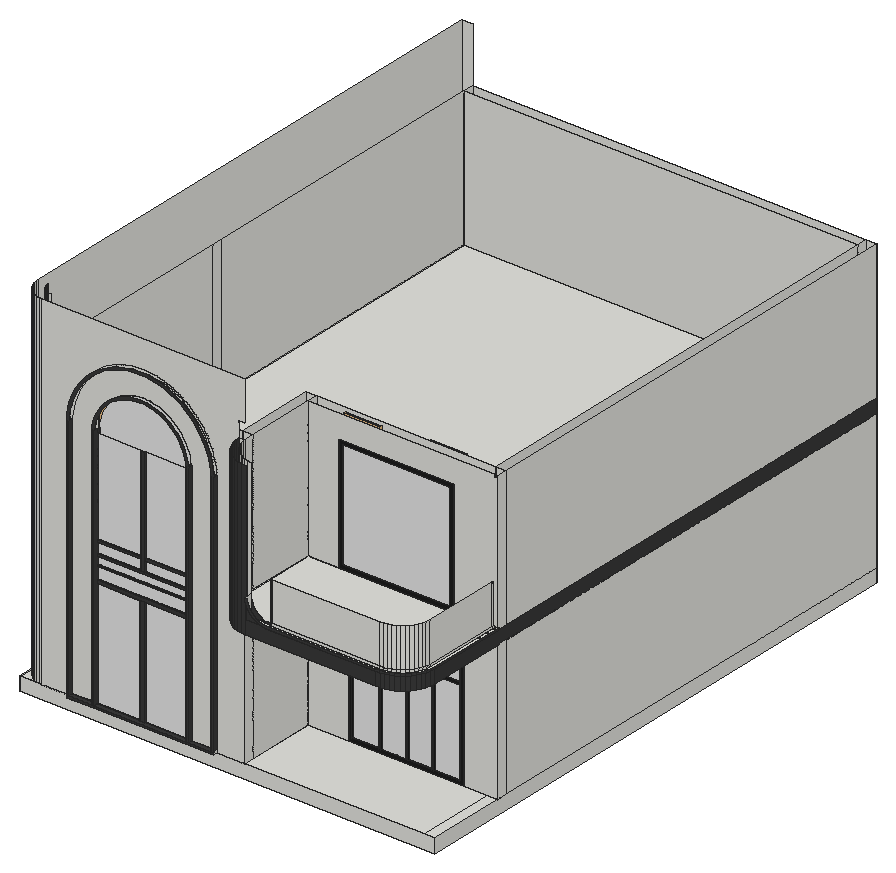
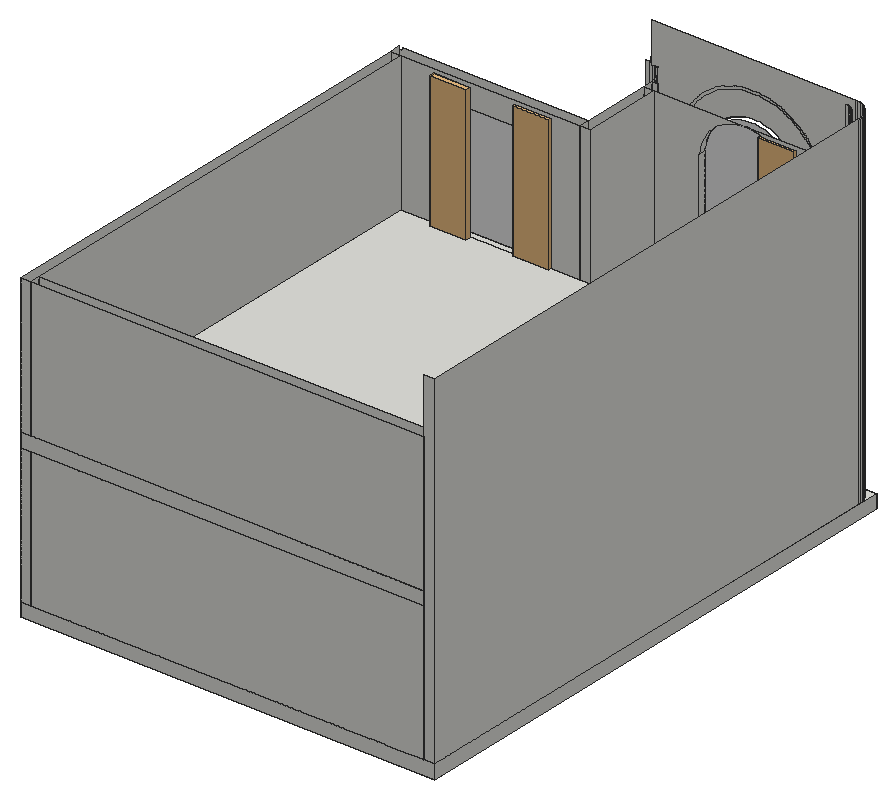
# SketchUp Ruby script. Lengths in inches.
U = 1.inch
M = Sketchup.active_model
def pt(a) = Geom::Point3d.new(a.map { |v| v * U })
def face(e, loops, mat)
  f = e.add_face(loops[0].map { |a| pt(a) })
  loops[1..].each { |l| e.add_face(l.map { |a| pt(a) }).erase! }
  f.material = f.back_material = mat if mat
  f
end
# faces: each face lists its corners as indices into pts; further lists are holes
def faces(e, pts, list, mat = nil) = list.each { |f| face(e, (f[0].is_a?(Array) ? f : [f]).map { |l| l.map { |i| pts[i] } }, mat) }
# xy, xz, yz: faces in a plane at the given z, y or x. An outline is a flat list of corners, or four numbers for a rectangle; further outlines are holes
def ring(l) = l.size == 4 ? [[l[0], l[1]], [l[2], l[1]], [l[2], l[3]], [l[0], l[3]]] : l.each_slice(2).to_a
def flat(e, list, mat, &to3) = list.each { |f| face(e, (f[0].is_a?(Array) ? f : [f]).map { |l| ring(l).map { |u, v| to3.(u, v) } }, mat) }
def xy(e, z, list, mat = nil) = flat(e, list, mat) { |x, y| [x, y, z] }
def xz(e, y, list, mat = nil) = flat(e, list, mat) { |x, z| [x, y, z] }
def yz(e, x, list, mat = nil) = flat(e, list, mat) { |y, z| [x, y, z] }
def lines(e, pts, list) = list.each { |a, b| e.add_line(pt(pts[a]), pt(pts[b])) }
# prism: a flat outline (further loops are holes) pulled along v
def prism(e, loops, v, mat = nil)
  f = face(e, loops, mat); d = Geom::Vector3d.new(v.map { |x| x * U })
  f.pushpull(f.normal.samedirection?(d) ? d.length : -d.length)
end
def box(e, o, s, mat = nil) = prism(e, [[o, [o[0] + s[0], o[1], o[2]], [o[0] + s[0], o[1] + s[1], o[2]], [o[0], o[1] + s[1], o[2]]]], [0, 0, s[2]], mat)
def at(x, y, z, deg = 0) = Geom::Transformation.translation(pt([x, y, z])) * Geom::Transformation.rotation(ORIGIN, Z_AXIS, deg.degrees)
def axes(o, x, y, z) = Geom::Transformation.new([*x, 0, *y, 0, *z, 0, *pt(o).to_a, 1])
def part(name) = M.definitions.add(name)
# library, detail: a bought-in or finely detailed component or shape, given as its bounding box
def library(name, o, s) = part(name).tap { |d| box(d.entities, o, s) }
def detail(e, o, s) = box(e.add_group.entities, o, s)
def put(e, d, t, mat = nil) = e.add_instance(d, t).tap { |i| i.material = mat if mat }
def group(e, t, mat = nil) = e.add_group.tap { |g| g.transformation = t; g.material = mat if mat }.entities
root = M.entities
M.materials.add("[Color M07]").color = [58, 58, 58]
M.materials.add("[Color M08]").color = [30, 30, 30]
M.materials.add("[Mirror 02]").color = [229, 229, 229]
c1 = library("Curtains 004",[-15.59,-2.26,0],[31.18,4.52,116.91])
xy(root,-12,[[0,27.75,360,507.75]])
xy(root,0,[[0,27.75,9,27.75,9,30.61,7.42,31.67,5.55,33.3,3.92,35.17,2.54,37.23,1.44,39.45,0.65,41.8,0.16,44.23,0,46.71],[18.96,27.75,195,27.75,195,36.75,18.96,36.75,17.66,36.84,16.38,37.09,15.15,37.51,13.98,38.08,12.9,38.81,11.92,39.67,11.06,40.65,10.33,41.73,9.76,42.9,9.34,44.13,9.09,45.41,9,46.71,9,30.61,9.48,30.29,11.7,29.19,14.05,28.4,16.48,27.91],[9,27.75,18.96,27.75,16.48,27.91,14.05,28.4,11.7,29.19,9.48,30.29,9,30.61],[195,27.75,351,96.75],[351,27.75,360,96.75],
  [9,30.61,7.42,31.67,5.55,33.3,3.92,35.17,2.54,37.23,1.44,39.45,0.65,41.8,0.16,44.23,0,46.71,0,507.75,9,507.75],[18.96,36.75,186,36.75,186,105.75,351,105.75,351,225.75,9,225.75,9,46.71,9.09,45.41,9.34,44.13,9.76,42.9,10.33,41.73,11.06,40.65,11.92,39.67,12.9,38.81,13.98,38.08,15.15,37.51,16.38,37.09,17.66,36.84],[186,36.75,195,105.75],[186,36.75,195,105.75],[195,96.75,229.97,105.75],
  [329.97,96.75,351,105.75],[351,96.75,360,105.75],[229.97,99.875,329.97,105.75],[351,105.75,360,507.75],[9,225.75,351,234.75],
  [9,234.75,351,498.75],[9,498.75,351,507.75]])
xy(root,0,[[42.96,24.0625,66.96,27.75],[66.96,24.0625,147,27.75],[147,24.0625,171,27.75]],"[Color M07]")
xy(root,0,[[229.97,96.75,329.97,97.5625],[229.97,97.5625,329.97,99.875]],"[Color M08]")
xy(root,2.17,[[42.96,24.0625,45.02,27.75],[64.9,24.0625,66.96,27.75],[147,24.0625,149.06,27.75],[168.94,24.0625,171,27.75],[66.96,29.9375,147,36.75]])
xy(root,2.17,[[45.02,24.0625,64.9,27.75],[66.96,24.0625,147,24.0625,147,27.75,108.98,27.75,108.98,26.6875,105.13,26.6875,105.13,27.75,66.96,27.75],[149.06,24.0625,168.94,27.75],[105.13,26.6875,108.98,27.75],[66.96,27.75,147,29.9375]],"[Color M07]")
xy(root,2.95,[[256.55,96.75,258.55,97.5625],[279.55,96.75,281.55,97.5625],[302.56,96.75,304.56,97.5625]])
xy(root,2.95,[[232.93,96.75,256.55,97.5625],[258.55,96.75,279.55,97.5625],[281.55,96.75,302.56,97.5625],[304.56,96.75,327.02,97.5625]],"[Color M08]")
xy(root,60.15,[[258.55,96.75,279.55,97.5625]])
xy(root,62.15,[[258.55,96.75,279.55,97.5625]],"[Color M08]")
xy(root,77.62,[[232.93,96.75,256.55,97.5625],[304.56,96.75,327.02,97.5625]])
xy(root,79.62,[[232.93,96.75,256.55,97.5625],[304.56,96.75,327.02,97.5625]],"[Color M08]")
xy(root,96.08,[[105.13,26.6875,108.98,27.75]])
xy(root,96.08,[[66.96,26.6875,105.13,27.75],[108.98,26.6875,147,27.75]],"[Color M07]")
xy(root,97.05,[[232.93,96.75,256.55,97.5625],[256.55,96.75,258.55,97.5625],[258.55,96.75,279.55,97.5625],[279.55,96.75,281.55,97.5625],[281.55,96.75,302.56,97.5625],
  [302.56,96.75,304.56,97.5625],[304.56,96.75,327.02,97.5625]])
xy(root,98.96,[[66.96,26.6875,147,27.75]],"[Color M07]")
xy(root,100,[[229.97,99.875,329.97,105.75]])
xy(root,100,[[229.97,96.75,329.97,97.5625],[229.97,97.5625,329.97,99.875]],"[Color M08]")
xy(root,109.4375,[[66.96,26.6875,147,27.75]],"[Color M07]")
xy(root,110.81,[[66.96,26.6875,147,27.75]],"[Color M07]")
xy(root,117.6875,[[66.96,26.6875,147,27.75]],"[Color M07]")
xy(root,119.24,[[105.32,26.6875,108.92,27.75]])
xy(root,119.24,[[66.96,26.6875,105.32,27.75],[108.92,26.6875,147,27.75]],"[Color M07]")
xy(root,120,[[[217.25,0.75,213.7,0.98,210.21,1.67,206.83,2.79,203.63,4.35,200.66,6.3,197.96,8.625,195.58,11.27,193.57,14.21,191.95,17.375,190.75,20.73,189.99,24.2,189.6875,27.75,195,27.75,195,96.75,360,96.75,360,27.6875,359.47,24.09,358.5,20.58,357.11,17.21,355.31,14.05,353.13,11.13,350.61,8.51,347.78,6.21,344.69,4.29,341.39,2.76,337.92,1.65,334.35,0.98,330.71,0.75],[206.46,76.4,339.34,83.03]],[9,36.75,9,225.75,351,225.75,351,105.75,186,105.75,186,36.75],[186,36.75,195,105.75],[195,96.75,351,105.75],[351,96.75,360,105.75],
  [351,105.75,360,507.75],[9,225.75,351,234.75],[9,234.75,351,498.75],[9,498.75,351,507.75]])
xy(root,124.5,[[206.46,76.4,339.34,83.03]])
xy(root,128.5625,[[66.96,26.6875,105.32,27.75],[108.92,26.6875,147,27.75]],"[Color M07]")
xy(root,130.14,[[66.96,26.6875,105.32,27.75]],"[Color M07]")
xy(root,130.37,[[108.92,26.6875,147,27.75]],"[Color M07]")
xy(root,132,[[217.25,0.75,235.85,6.3],[235.85,4.75,235.85,5.39,330.57,5.39,333.77,5.59,336.78,6.16,339.7,7.09,342.48,8.38,345.08,10,347.46,11.93,349.58,14.14,351.41,16.6,352.93,19.26,354.1,22.09,354.92,25.04,355.36,28.03,355.36,96.75,356,96.75,356,27.98,355.55,24.91,354.71,21.88,353.51,18.98,351.95,16.24,350.07,13.73,347.9,11.46,345.45,9.48,342.79,7.8125,339.93,6.49,336.94,5.53,333.85,4.95,330.59,4.75],[235.85,5.39,236.49,5.39,236.49,6.95,217.29,6.95,214.6,7.29,211.96,7.95,209.41,8.91,206.99,10.15,204.73,11.67,202.67,13.44,200.82,15.44,199.22,17.64,197.89,20.01,196.84,22.52,196.09,25.13,195.64,27.8,195.64,96.11,355.36,96.11,355.36,96.75,195,96.75,195,27.75,195.46,24.99,196.23,22.31,197.31,19.73,198.68,17.29,200.32,15.03,202.22,12.98,204.34,11.16,206.66,9.6,209.15,8.32,211.76,7.33,214.48,6.66,217.25,6.3,235.85,6.3],[236.49,5.39,330.57,5.39,333.77,5.59,336.78,6.16,339.7,7.09,342.48,8.38,345.08,10,347.46,11.93,349.58,14.14,351.41,16.6,352.93,19.26,354.1,22.09,354.92,25.04,355.36,28.03,355.36,96.11,195.64,96.11,195.64,27.8,196.09,25.13,196.84,22.52,197.89,20.01,199.22,17.64,200.82,15.44,202.67,13.44,204.73,11.67,206.99,10.15,209.41,8.91,211.96,7.95,214.6,7.29,217.29,6.95,236.49,6.95],[9,36.75,186,36.75,186,105.75,351,105.75,351,498.75,9,498.75],
  [186,36.75,195,105.75],[356,95.25,360,96.75],[195,96.75,221.4,105.75],[321.4,96.75,360,105.75],[221.4,99.875,321.4,105.75],
  [351,105.75,360,507.75],[9,498.75,351,507.75]])
xy(root,132,[[235.85,0,235.85,0.75,330.71,0.75,334.35,0.98,337.92,1.65,341.39,2.76,344.69,4.29,347.78,6.21,350.61,8.51,353.13,11.13,355.31,14.05,357.11,17.21,358.5,20.58,359.47,24.09,360,27.6875,360,95.25,360.75,95.25,360.75,27.63,360.21,23.93,359.21,20.33,357.78,16.88,355.9375,13.64,353.7,10.65,351.12,7.96,348.22,5.6,345.05,3.63,341.66,2.06,338.11,0.92,334.4375,0.23,330.74,0],[360,95.25,360.75,96.75]],"[Color M07]")
xy(root,132,[[221.4,96.75,321.4,97.5625],[221.4,97.5625,321.4,99.875]],"[Color M08]")
xz(root,0,[[235.85,132,330.74,132,330.74,133.9375,235.91,133.9375,233.52,134.1,231.24,134.59,229.05,135.38,227,136.47,225.11,137.84,223.43,139.45,221.99,141.28,220.82,143.3,219.9375,145.45,219.37,147.71,219.1875,149.34,217.25,149.34,217.25,149.24,217.26,149.16,217.35,148.3,217.46,147.37,217.67,146.52,218.09,144.85,219.08,142.44,220.38,140.19,221.99,138.15,223.86,136.35,225.97,134.82,228.27,133.61,230.71,132.72,233.25,132.18]],"[Color M07]")
xz(root,0.75,[[217.25,120,330.71,132],[217.25,132,235.85,132,233.25,132.18,230.71,132.72,228.27,133.61,225.97,134.82,223.86,136.35,221.99,138.15,220.38,140.19,219.08,142.44,218.09,144.85,217.67,146.52,217.46,147.37,217.43,147.62,217.26,149.16,217.25,149.24]],"[Color M07]")
xz(root,4.75,[[235.85,132,235.85,133.94,235.91,133.9375,330.59,133.9375,330.59,132]])
xz(root,4.75,[[235.85,132,233.25,132.18,230.71,132.72,228.27,133.61,227.63,133.94,235.85,133.94]],"[Color M07]")
xz(root,5.39,[[235.85,132,236.49,168],[236.49,132,330.57,168]])
xz(root,6.3,[[217.25,132,217.25,149.24,217.46,147.37,218.09,144.85,219.08,142.44,220.38,140.19,221.99,138.15,223.86,136.35,225.97,134.82,228.27,133.61,230.71,132.72,233.25,132.18,235.85,132]],"[Color M07]")
xz(root,24.0625,[[42.96,0,66.96,2.17],[66.96,0,147,2.17],[147,0,171,2.17],[42.96,2.17,45.02,2.17,45.02,215.89,45.49,220.52,46.32,225.12,47.49,229.64,49,234.07,50.83,238.37,52.99,242.52,55.45,246.49,58.2,250.27,61.23,253.83,64.52,257.15,68.05,260.22,71.8,263.01,75.74,265.51,79.87,267.71,84.15,269.59,88.56,271.14,93.07,272.36,97.66,273.24,102.31,273.76,106.98,273.9375,111.65,273.76,116.3,273.24,120.89,272.36,125.4,271.14,129.81,269.59,134.09,267.71,138.21,265.51,142.16,263.01,145.91,260.22,149.44,257.15,152.73,253.83,155.76,250.27,158.51,246.49,160.97,242.52,163.125,238.37,164.96,234.07,166.47,229.64,167.64,225.12,168.46,220.52,168.94,215.89,168.94,2.17,171,2.17,171,216,170.51,220.8,169.65,225.56,168.44,230.23,166.89,234.81,164.99,239.25,162.76,243.53,160.22,247.64,157.375,251.54,154.25,255.22,150.85,258.66,147.2,261.82,143.33,264.71,139.25,267.29,134.99,269.5625,130.57,271.51,126.01,273.11,121.35,274.37,116.6,275.27,111.81,275.82,106.98,276,102.15,275.82,97.35,275.27,92.61,274.37,87.95,273.11,83.39,271.51,78.97,269.5625,74.71,267.29,70.63,264.71,66.75,261.82,63.11,258.66,59.71,255.22,56.58,251.54,53.74,247.64,51.2,243.53,48.97,239.25,47.07,234.81,45.52,230.23,44.31,225.56,43.45,220.8,42.96,216],[64.9,2.17,66.96,2.17,66.96,216,67.375,218.92,68.01,221.8,68.85,224.62,69.89,227.38,71.13,230.05,72.57,232.625,74.1875,235.09,75.98,237.43,77.95,239.625,80.0625,241.68,82.33,243.57,84.72,245.28,87.23,246.82,89.85,248.17,92.57,249.33,95.35,250.28,98.21,251.03,101.1,251.57,104.03,251.89,106.98,252,109.92,251.89,112.85,251.57,115.75,251.03,118.6,250.28,121.39,249.33,124.1,248.17,126.72,246.82,129.24,245.28,131.63,243.57,133.89,241.68,136.01,239.625,137.97,237.43,139.77,235.09,141.39,232.625,142.82,230.05,144.07,227.38,145.11,224.62,145.95,221.8,146.58,218.92,147,216,147,2.17,149.06,2.17,149.06,216.15,148.61,219.28,147.95,222.3125,147.06,225.28,145.97,228.18,144.66,230.99,143.15,233.69,141.45,236.28,139.5625,238.74,137.5,241.05,135.27,243.21,132.89,245.19,130.38,247,127.74,248.62,124.98,250.04,122.13,251.25,119.2,252.26,116.2,253.04,113.16,253.61,110.08,253.95,106.98,254.0625,103.88,253.95,100.8,253.61,97.76,253.04,94.76,252.26,91.83,251.25,88.98,250.04,86.22,248.62,83.58,247,81.0625,245.19,78.6875,243.21,76.46,241.05,74.4,238.74,72.51,236.28,70.81,233.69,69.3,230.99,67.99,228.18,66.89,225.28,66.01,222.3125,65.35,219.28,64.9,216.15]],"[Color M07]")
xz(root,26.6875,[[105.13,2.17,108.98,96.08],[66.96,96.08,147,98.96],[66.96,109.4375,147,110.81],[66.96,117.6875,147,119.24],[105.32,119.24,108.92,212.44],
  [66.96,128.5625,105.32,130.14],[108.92,128.5625,147,130.37]],"[Color M07]")
xz(root,27.75,[[0,-12,360,0],[18.96,0,42.96,0,42.96,216,43.45,220.8,44.31,225.56,45.52,230.23,47.07,234.81,48.97,239.25,51.2,243.53,53.74,247.64,56.58,251.54,59.71,255.22,63.11,258.66,66.75,261.82,70.63,264.71,74.71,267.29,78.97,269.5625,83.39,271.51,87.95,273.11,92.61,274.37,97.35,275.27,102.15,275.82,106.98,276,111.81,275.82,116.6,275.27,121.35,274.37,126.01,273.11,130.57,271.51,134.99,269.5625,139.25,267.29,143.33,264.71,147.2,261.82,150.85,258.66,154.25,255.22,157.375,251.54,160.22,247.64,162.76,243.53,164.99,239.25,166.89,234.81,168.44,230.23,169.65,225.56,170.51,220.8,171,216,171,0,195,0,195,120,189.6875,120,189.6875,264,189.25,264,189.25,265.57,195,265.57,195,300,18.96,300],[42.96,0,66.96,2.17],[66.96,0,147,2.17],[147,0,171,2.17],
  [42.96,2.17,42.96,216,43.45,220.8,44.31,225.56,45.52,230.23,47.07,234.81,48.97,239.25,51.2,243.53,53.74,247.64,56.58,251.54,59.71,255.22,63.11,258.66,66.75,261.82,70.63,264.71,74.71,267.29,78.97,269.5625,83.39,271.51,87.95,273.11,92.61,274.37,97.35,275.27,102.15,275.82,106.98,276,111.81,275.82,116.6,275.27,121.35,274.37,126.01,273.11,130.57,271.51,134.99,269.5625,139.25,267.29,143.33,264.71,147.2,261.82,150.85,258.66,154.25,255.22,157.375,251.54,160.22,247.64,162.76,243.53,164.99,239.25,166.89,234.81,168.44,230.23,169.65,225.56,170.51,220.8,171,216,171,2.17,168.94,2.17,168.94,215.89,168.46,220.52,167.64,225.12,166.47,229.64,164.96,234.07,163.125,238.37,160.97,242.52,158.51,246.49,155.76,250.27,152.73,253.83,149.44,257.15,145.91,260.22,142.16,263.01,138.21,265.51,134.09,267.71,129.81,269.59,125.4,271.14,120.89,272.36,116.3,273.24,111.65,273.76,106.98,273.9375,102.31,273.76,97.66,273.24,93.07,272.36,88.56,271.14,84.15,269.59,79.87,267.71,75.74,265.51,71.8,263.01,68.05,260.22,64.52,257.15,61.23,253.83,58.2,250.27,55.45,246.49,52.99,242.52,50.83,238.37,49,234.07,47.49,229.64,46.32,225.12,45.49,220.52,45.02,215.89,45.02,2.17],[45.02,2.17,64.9,2.17,64.9,216.15,65.35,219.28,66.01,222.3125,66.89,225.28,67.99,228.18,69.3,230.99,70.81,233.69,72.51,236.28,74.4,238.74,76.46,241.05,78.6875,243.21,81.0625,245.19,83.58,247,86.22,248.62,88.98,250.04,91.83,251.25,94.76,252.26,97.76,253.04,100.8,253.61,103.88,253.95,106.98,254.0625,110.08,253.95,113.16,253.61,116.2,253.04,119.2,252.26,122.13,251.25,124.98,250.04,127.74,248.62,130.38,247,132.89,245.19,135.27,243.21,137.5,241.05,139.5625,238.74,141.45,236.28,143.15,233.69,144.66,230.99,145.97,228.18,147.06,225.28,147.95,222.3125,148.61,219.28,149.06,216.15,149.06,2.17,168.94,2.17,168.94,215.89,168.46,220.52,167.64,225.12,166.47,229.64,164.96,234.07,163.125,238.37,160.97,242.52,158.51,246.49,155.76,250.27,152.73,253.83,149.44,257.15,145.91,260.22,142.16,263.01,138.21,265.51,134.09,267.71,129.81,269.59,125.4,271.14,120.89,272.36,116.3,273.24,111.65,273.76,106.98,273.9375,102.31,273.76,97.66,273.24,93.07,272.36,88.56,271.14,84.15,269.59,79.87,267.71,75.74,265.51,71.8,263.01,68.05,260.22,64.52,257.15,61.23,253.83,58.2,250.27,55.45,246.49,52.99,242.52,50.83,238.37,49,234.07,47.49,229.64,46.32,225.12,45.49,220.52,45.02,215.89],[105.13,2.17,108.98,96.08],[66.96,96.08,147,98.96],[66.96,109.4375,147,110.81],
  [66.96,117.6875,147,119.24],[105.32,119.24,108.92,212.44],[189.6875,120,195,252],[66.96,128.5625,105.32,130.14],[108.92,128.5625,147,130.37]])
xz(root,27.75,[[66.96,2.17,105.13,96.08],[108.98,2.17,147,96.08],[66.96,98.96,147,109.4375],[66.96,110.81,147,117.6875],[66.96,119.24,105.32,128.5625],
  [108.92,119.24,147,128.5625],[66.96,130.14,105.32,212.44],[108.92,130.37,147,212.44]],"[Mirror 02]")
xz(root,29.9375,[[66.96,2.17,66.96,216,67.375,218.92,68.01,221.8,68.85,224.62,69.89,227.38,71.13,230.05,72.57,232.625,74.1875,235.09,75.98,237.43,77.95,239.625,80.0625,241.68,82.33,243.57,84.72,245.28,87.23,246.82,89.85,248.17,92.57,249.33,95.35,250.28,98.21,251.03,101.1,251.57,104.03,251.89,106.98,252,109.92,251.89,112.85,251.57,115.75,251.03,118.6,250.28,121.39,249.33,124.1,248.17,126.72,246.82,129.24,245.28,131.63,243.57,133.89,241.68,136.01,239.625,137.97,237.43,139.77,235.09,141.39,232.625,142.82,230.05,144.07,227.38,145.11,224.62,145.95,221.8,146.58,218.92,147,216,147,2.17]],"[Mirror 02]")
xz(root,36.75,[[18.96,0,18.96,120,66.96,120,66.96,2.17,147,2.17,147,120,186,120,186,0],[186,0,195,120],[9,120,18.96,132],[18.96,120,66.96,132],[66.96,120,147,132],
  [147,120,186,132],[186,120,195,132],[18.96,132,18.96,252,106.98,252,104.03,251.89,101.1,251.57,98.21,251.03,95.35,250.28,92.57,249.33,89.85,248.17,87.23,246.82,84.72,245.28,82.33,243.57,80.0625,241.68,77.95,239.625,75.98,237.43,74.1875,235.09,72.57,232.625,71.13,230.05,69.89,227.38,68.85,224.62,68.01,221.8,67.375,218.92,66.96,216,66.96,132],[147,132,147,216,146.58,218.92,145.95,221.8,145.11,224.62,144.07,227.38,142.82,230.05,141.39,232.625,139.77,235.09,137.97,237.43,136.01,239.625,133.89,241.68,131.63,243.57,129.24,245.28,126.72,246.82,124.1,248.17,121.39,249.33,118.6,250.28,115.75,251.03,112.85,251.57,109.92,251.89,106.98,252,186,252,186,132],[186,132,195,252]])
xz(root,76.4,[[206.46,120,339.34,124.5]])
xz(root,83.03,[[206.46,120,339.34,124.5]])
xz(root,96.75,[[195,0,229.97,0,229.97,100,329.97,100,329.97,0,360,0,360,120,195,120],[195,132,221.4,132,221.4,232,321.4,232,321.4,132,355.36,132,355.36,168,356,168,356,133.9375,360,133.9375,360,250.0625,356,250.0625,356,252,195,252],[355.36,132,356,168],[356,132,360,133.9375],[360,132,360.75,133.9375]])
xz(root,96.75,[[[229.97,0,329.97,100],[232.93,2.95,327.02,97.05]],[256.55,2.95,258.55,97.05],[279.55,2.95,281.55,97.05],[302.56,2.95,304.56,97.05],[258.55,60.15,279.55,62.15],
  [232.93,77.62,256.55,79.62],[304.56,77.62,327.02,79.62],[[221.4,132,321.4,232],[224.36,134.95,318.45,229.05]]],"[Color M08]")
xz(root,97.5625,[[[229.97,0,329.97,100],[232.93,2.95,327.02,97.05]],[256.55,2.95,258.55,97.05],[279.55,2.95,281.55,97.05],[302.56,2.95,304.56,97.05],[258.55,60.15,279.55,62.15],
  [232.93,77.62,256.55,79.62],[304.56,77.62,327.02,79.62],[[221.4,132,321.4,232],[224.36,134.95,318.45,229.05]]])
xz(root,97.5625,[[232.93,2.95,256.55,77.62],[258.55,2.95,279.55,60.15],[281.55,2.95,302.56,97.05],[304.56,2.95,327.02,77.62],[258.55,62.15,279.55,97.05],
  [232.93,79.62,256.55,97.05],[304.56,79.62,327.02,97.05]],"[Mirror 02]")
xz(root,99.875,[[229.97,0,329.97,100],[221.4,132,321.4,232]],"[Mirror 02]")
xz(root,105.75,[[186,0,195,120],[195,0,195,120,351,120,351,0,329.97,0,329.97,100,229.97,100,229.97,0],[351,0,360,120],[186,132,195,252],[195,132,195,252,351,252,351,132,321.4,132,321.4,232,221.4,232,221.4,132],
  [351,132,360,252]])
xz(root,225.75,[[9,0,351,120]])
xz(root,234.75,[[9,0,351,120]])
xz(root,498.75,[[9,0,351,120],[9,132,351,252]])
xz(root,507.75,[[0,-12,360,0],[0,0,9,300],[9,0,351,120],[351,0,360,120],[9,120,360,132],
  [9,132,351,252],[351,132,360,252]])
yz(root,0,[[27.75,-12,507.75,0],[46.71,0,507.75,300]])
yz(root,9,[[46.71,0,225.75,120],[225.75,0,234.75,120],[234.75,0,498.75,120],[498.75,0,507.75,120],[36.75,120,46.71,132],
  [46.71,120,225.75,132],[225.75,120,234.75,132],[234.75,120,498.75,132],[498.75,120,507.75,132],[46.71,132,225.75,252],
  [225.75,132,234.75,252],[234.75,132,498.75,252],[498.75,132,507.75,252]])
yz(root,42.96,[[24.0625,0,27.75,2.17],[24.0625,2.17,27.75,216]],"[Color M07]")
yz(root,45.02,[[24.0625,2.17,27.75,215.89]],"[Color M07]")
yz(root,64.9,[[24.0625,2.17,27.75,216.15]],"[Color M07]")
yz(root,66.96,[[24.0625,0,27.75,2.17],[29.9375,2.17,36.75,216]])
yz(root,66.96,[[24.0625,2.17,27.75,2.17,27.75,96.08,26.6875,96.08,26.6875,98.96,27.75,98.96,27.75,109.4375,26.6875,109.4375,26.6875,110.81,27.75,110.81,27.75,117.6875,26.6875,117.6875,26.6875,119.24,27.75,119.24,27.75,128.5625,26.6875,128.5625,26.6875,130.14,27.75,130.14,27.75,212.44,26.6875,212.44,26.6875,216,24.0625,216],[27.75,2.17,29.9375,216],[26.6875,96.08,27.75,98.96],[26.6875,109.4375,27.75,110.81],[26.6875,117.6875,27.75,119.24],
  [26.6875,128.5625,27.75,130.14]],"[Color M07]")
yz(root,105.13,[[26.6875,2.17,27.75,96.08]],"[Color M07]")
yz(root,105.32,[[26.6875,128.5625,27.75,130.14]])
yz(root,105.32,[[26.6875,119.24,27.75,128.5625],[26.6875,130.14,27.75,212.44]],"[Color M07]")
yz(root,108.92,[[26.6875,128.5625,27.75,130.37]])
yz(root,108.92,[[26.6875,119.24,27.75,128.5625],[26.6875,130.37,27.75,212.44]],"[Color M07]")
yz(root,108.98,[[26.6875,2.17,27.75,96.08]],"[Color M07]")
yz(root,147,[[24.0625,0,27.75,2.17],[29.9375,2.17,36.75,216]])
yz(root,147,[[24.0625,2.17,24.0625,216,26.6875,216,26.6875,212.44,27.75,212.44,27.75,130.37,26.6875,130.37,26.6875,128.5625,27.75,128.5625,27.75,119.24,26.6875,119.24,26.6875,117.6875,27.75,117.6875,27.75,110.81,26.6875,110.81,26.6875,109.4375,27.75,109.4375,27.75,98.96,26.6875,98.96,26.6875,96.08,27.75,96.08,27.75,2.17],[27.75,2.17,29.9375,216],[26.6875,96.08,27.75,98.96],[26.6875,109.4375,27.75,110.81],[26.6875,117.6875,27.75,119.24],
  [26.6875,128.5625,27.75,130.37]],"[Color M07]")
yz(root,149.06,[[24.0625,2.17,27.75,216.15]],"[Color M07]")
yz(root,168.94,[[24.0625,2.17,27.75,215.89]],"[Color M07]")
yz(root,171,[[24.0625,0,27.75,2.17]])
yz(root,171,[[24.0625,2.17,27.75,216]],"[Color M07]")
yz(root,186,[[36.75,0,105.75,120],[36.75,132,105.75,252]])
yz(root,195,[[27.75,0,36.75,120],[36.75,0,96.75,120],[96.75,0,105.75,120],[27.75,120,36.75,132],[27.75,132,36.75,252],
  [36.75,132,96.75,252],[96.75,132,105.75,252]])
yz(root,206.46,[[76.4,120,83.03,124.5]])
yz(root,217.25,[[0.75,132,6.3,149.24]])
yz(root,221.4,[[99.875,132,105.75,232]])
yz(root,221.4,[[96.75,132,97.5625,232],[97.5625,132,99.875,232]],"[Color M08]")
yz(root,229.97,[[99.875,0,105.75,100]])
yz(root,229.97,[[96.75,0,97.5625,100],[97.5625,0,99.875,100]],"[Color M08]")
yz(root,232.93,[[96.75,77.62,97.5625,79.62]])
yz(root,232.93,[[96.75,2.95,97.5625,77.62],[96.75,79.62,97.5625,97.05]],"[Color M08]")
yz(root,235.85,[[4.75,132,5.39,168]])
yz(root,256.55,[[96.75,77.62,97.5625,79.62]])
yz(root,256.55,[[96.75,2.95,97.5625,77.62],[96.75,79.62,97.5625,97.05]],"[Color M08]")
yz(root,258.55,[[96.75,60.15,97.5625,62.15]])
yz(root,258.55,[[96.75,2.95,97.5625,60.15],[96.75,62.15,97.5625,79.62],[96.75,79.62,97.5625,97.05]],"[Color M08]")
yz(root,279.55,[[96.75,60.15,97.5625,62.15]])
yz(root,279.55,[[96.75,2.95,97.5625,60.15],[96.75,62.15,97.5625,97.05]],"[Color M08]")
yz(root,281.55,[[96.75,2.95,97.5625,62.15],[96.75,62.15,97.5625,97.05]],"[Color M08]")
yz(root,302.56,[[96.75,2.95,97.5625,97.05]],"[Color M08]")
yz(root,304.56,[[96.75,77.62,97.5625,79.62]])
yz(root,304.56,[[96.75,2.95,97.5625,77.62],[96.75,79.62,97.5625,97.05]],"[Color M08]")
yz(root,321.4,[[99.875,132,105.75,232]])
yz(root,321.4,[[96.75,132,97.5625,232],[97.5625,132,99.875,232]],"[Color M08]")
yz(root,327.02,[[96.75,77.62,97.5625,79.62],[96.75,79.62,97.5625,97.05]])
yz(root,327.02,[[96.75,2.95,97.5625,77.62]],"[Color M08]")
yz(root,329.97,[[99.875,0,105.75,100]])
yz(root,329.97,[[96.75,0,97.5625,100],[97.5625,0,99.875,100]],"[Color M08]")
yz(root,339.34,[[76.4,120,83.03,124.5]])
yz(root,351,[[105.75,0,225.75,120],[225.75,0,234.75,120],[234.75,0,498.75,120],[498.75,0,507.75,120],[105.75,132,498.75,252],
  [498.75,132,507.75,252]])
yz(root,355.36,[[28.03,132,95.25,168],[95.25,132,96.11,168],[96.11,132,96.75,168]])
yz(root,356,[[27.98,132,95.25,133.9375],[95.25,132,96.75,133.9375]])
yz(root,360,[[27.75,-12,507.75,0],[96.75,0,105.75,120],[105.75,0,507.75,120],[96.75,132,105.75,252],[105.75,132,507.75,252]])
yz(root,360,[[27.6875,120,507.75,132]],"[Color M07]")
yz(root,360.75,[[27.63,132,95.25,133.9375],[95.25,132,96.75,133.9375]],"[Color M07]")
p = [[16.48,27.91,0],[18.96,27.75,0],[18.96,27.75,300],[16.48,27.91,300],[14.05,28.4,0],[14.05,28.4,300],
  [11.7,29.19,0],[11.7,29.19,300],[9.48,30.29,0],[9.48,30.29,300],[9,30.61,0],[9,30.61,300],
  [7.42,31.67,0],[7.42,31.67,300],[5.55,33.3,0],[5.55,33.3,300],[3.92,35.17,0],[3.92,35.17,300],
  [2.54,37.23,0],[2.54,37.23,300],[18.96,36.75,0],[17.66,36.84,0],[17.66,36.84,300],[18.96,36.75,300],
  [18.96,36.75,264],[18.96,36.75,252],[18.96,36.75,132],[18.96,36.75,120],[16.38,37.09,0],[16.38,37.09,300],
  [15.15,37.51,0],[15.15,37.51,300],[1.44,39.45,0],[1.44,39.45,300],[13.98,38.08,0],[13.98,38.08,300],
  [12.9,38.81,0],[12.9,38.81,300],[11.92,39.67,0],[11.92,39.67,300],[0.65,41.8,0],[0.65,41.8,300],
  [11.06,40.65,0],[11.06,40.65,300],[10.33,41.73,0],[10.33,41.73,300],[9.76,42.9,0],[9.76,42.9,300],
  [0.16,44.23,0],[0.16,44.23,300],[9.34,44.13,0],[9.34,44.13,300],[9.09,45.41,0],[9.09,45.41,300],
  [0,46.71,0],[0.02,46.41,300],[0,46.71,300],[9,46.71,0],[9,46.71,120],[9,46.71,132],
  [9,46.71,252],[9,46.71,264],[9,46.71,300],[217.25,0.75,120],[217.25,0.75,132],[217.25,0.75,149.24],
  [217.25,0.75,149.34],[217.25,0.75,238.1],[217.25,0.75,238.34],[217.25,0.75,252],[213.7,0.98,252],[213.7,0.98,120],
  [334.35,0.98,132],[330.71,0.75,132],[330.71,0.75,120],[334.35,0.98,120],[210.21,1.67,252],[210.21,1.67,120],
  [337.92,1.65,132],[337.92,1.65,120],[341.39,2.76,132],[341.39,2.76,120],[206.83,2.79,252],[206.83,2.79,120],
  [203.63,4.35,252],[203.63,4.35,120],[344.69,4.29,132],[344.69,4.29,120],[200.66,6.3,252],[200.66,6.3,120],
  [347.78,6.21,132],[347.78,6.21,120],[350.61,8.51,132],[350.61,8.51,120],[197.96,8.625,252],[197.96,8.625,120],
  [353.13,11.13,132],[353.13,11.13,120],[195.58,11.27,252],[195.58,11.27,120],[355.31,14.05,132],[355.31,14.05,120],
  [193.57,14.21,252],[193.57,14.21,120],[357.11,17.21,132],[357.11,17.21,120],[191.95,17.375,252],[191.95,17.375,120],
  [358.5,20.58,132],[358.5,20.58,120],[190.75,20.73,252],[190.75,20.73,120],[359.47,24.09,132],[359.47,24.09,120],
  [189.99,24.2,252],[189.99,24.2,120],[360,27.6875,132],[360,27.6875,120],[189.6875,27.75,252],[189.6875,27.75,120],
  [233.25,0,132.18],[233.25,0.75,132.18],[235.85,0.75,132],[235.85,0,132],[334.4375,0.23,132],[334.4375,0.23,133.9375],
  [330.74,0,133.9375],[330.74,0,132],[338.11,0.92,132],[338.11,0.92,133.9375],[341.66,2.06,132],[341.66,2.06,133.9375],
  [345.05,3.63,132],[345.05,3.63,133.9375],[348.22,5.6,132],[348.22,5.6,133.9375],[235.85,4.75,132],[235.85,5.39,132],
  [235.85,6.3,132],[233.25,6.3,132.18],[233.25,4.75,132.18],[333.85,4.95,132],[333.85,4.95,133.9375],[330.59,4.75,133.9375],
  [330.59,4.75,132],[336.94,5.53,132],[336.94,5.53,133.9375],[333.77,5.59,132],[330.57,5.39,132],[330.57,5.39,168],
  [333.77,5.59,168],[339.93,6.49,132],[339.93,6.49,133.9375],[336.78,6.16,132],[336.78,6.16,168],[351.12,7.96,132],
  [351.12,7.96,133.9375],[339.7,7.09,132],[339.7,7.09,168],[217.25,6.3,132],[214.48,6.66,132],[214.48,6.66,252],
  [217.25,6.3,252],[217.25,6.3,238.34],[217.25,6.3,149.24],[342.79,7.8125,132],[342.79,7.8125,133.9375],[211.76,7.33,132],
  [211.76,7.33,252],[342.48,8.38,132],[342.48,8.38,168],[209.15,8.32,132],[209.15,8.32,252],[345.45,9.48,132],
  [345.45,9.48,133.9375],[353.7,10.65,132],[353.7,10.65,133.9375],[206.66,9.6,132],[206.66,9.6,252],[345.08,10,132],
  [345.08,10,168],[347.9,11.46,132],[347.9,11.46,133.9375],[204.34,11.16,132],[204.34,11.16,252],[347.46,11.93,132],
  [347.46,11.93,168],[355.9375,13.64,132],[355.9375,13.64,133.9375],[202.22,12.98,132],[202.22,12.98,252],[350.07,13.73,132],
  [350.07,13.73,133.9375],[349.58,14.14,132],[349.58,14.14,168],[200.32,15.03,132],[200.32,15.03,252],[357.78,16.88,132],
  [357.78,16.88,133.9375],[351.95,16.24,132],[351.95,16.24,133.9375],[351.41,16.6,132],[351.41,16.6,168],[198.68,17.29,132],
  [198.68,17.29,252],[353.51,18.98,132],[353.51,18.98,133.9375],[352.93,19.26,132],[352.93,19.26,168],[359.21,20.33,132],
  [359.21,20.33,133.9375],[197.31,19.73,132],[197.31,19.73,252],[354.71,21.88,132],[354.71,21.88,133.9375],[354.1,22.09,132],
  [354.1,22.09,168],[196.23,22.31,132],[196.23,22.31,252],[360.21,23.93,132],[360.21,23.93,133.9375],[355.55,24.91,132],
  [355.55,24.91,133.9375],[354.92,25.04,132],[354.92,25.04,168],[195.46,24.99,132],[195.46,24.99,252],[360.75,27.63,132],
  [360.75,27.63,133.9375],[356,27.98,132],[356,27.98,133.9375],[195,27.75,132],[195,27.75,252],[355.36,28.03,132],
  [355.36,28.03,168],[230.71,0,132.72],[230.71,0.75,132.72],[230.71,6.3,132.72],[230.71,4.75,132.72]]
faces(root,p,[[0,1,2,3],[4,0,3,5],[6,4,5,7],[8,6,7,9],[10,8,9,11],[12,10,11,13],[14,12,13,15],[16,14,15,17],
  [18,16,17,19],[20,21,22,23,24,25,26,27],[21,28,29,22],[28,30,31,29],[32,18,19,33],[30,34,35,31],[34,36,37,35],[36,38,39,37],
  [40,32,33,41],[38,42,43,39],[42,44,45,43],[44,46,47,45],[48,40,41,49],[46,50,51,47],[50,52,53,51],[54,48,49,55,56],
  [52,57,58,59,60,61,62,53],[141,142,143,144],[145,146,142,141],[147,148,149,150],[151,152,146,145],[153,147,150,154],[157,153,154,158],[159,160,161,162,163,164],
  [165,166,152,151],[160,167,168,161],[169,157,158,170],[167,171,172,168],[173,174,166,165],[171,177,178,172],[179,169,170,180],[181,182,174,173],
  [177,183,184,178],[185,179,180,186],[183,189,190,184],[191,192,182,181],[193,185,186,194],[189,195,196,190],[199,200,192,191],[201,193,194,202],
  [195,203,204,196],[205,206,200,199],[207,201,202,208],[203,211,212,204],[213,214,206,205],[215,207,208,216],[211,217,218,212],[221,222,214,213],
  [223,215,216,224],[217,225,226,218],[229,230,222,221],[225,231,232,226],[233,223,224,234]])
faces(root,p,[[63,64,65,66,67,68,69,70,71],[72,73,74,75],[71,70,76,77],[78,72,75,79],[80,78,79,81],[77,76,82,83],[83,82,84,85],[86,80,81,87],
  [85,84,88,89],[90,86,87,91],[92,90,91,93],[89,88,94,95],[96,92,93,97],[95,94,98,99],[100,96,97,101],[99,98,102,103],
  [104,100,101,105],[103,102,106,107],[108,104,105,109],[107,106,110,111],[112,108,109,113],[111,110,114,115],[116,112,113,117],[115,114,118,119],
  [120,121,122,123],[124,125,126,127],[128,129,125,124],[130,131,129,128],[132,133,131,130],[134,135,133,132],[136,137,138,139,140],[155,156,135,134],
  [175,176,156,155],[187,188,176,175],[197,198,188,187],[209,210,198,197],[219,220,210,209],[227,228,220,219],[121,120,235,236],[140,139,237,238]],"[Color M07]")
put(root,c1,at(245.39,105.75,0))
put(root,c1,at(314.5625,105.75,0))
put(root,c1,at(80.74,36.75,2.17))
put(root,c1,at(78.48,36.75,132))
put(root,c1,at(236.4,105.75,132))
put(root,c1,at(305.62,108.78,132))
